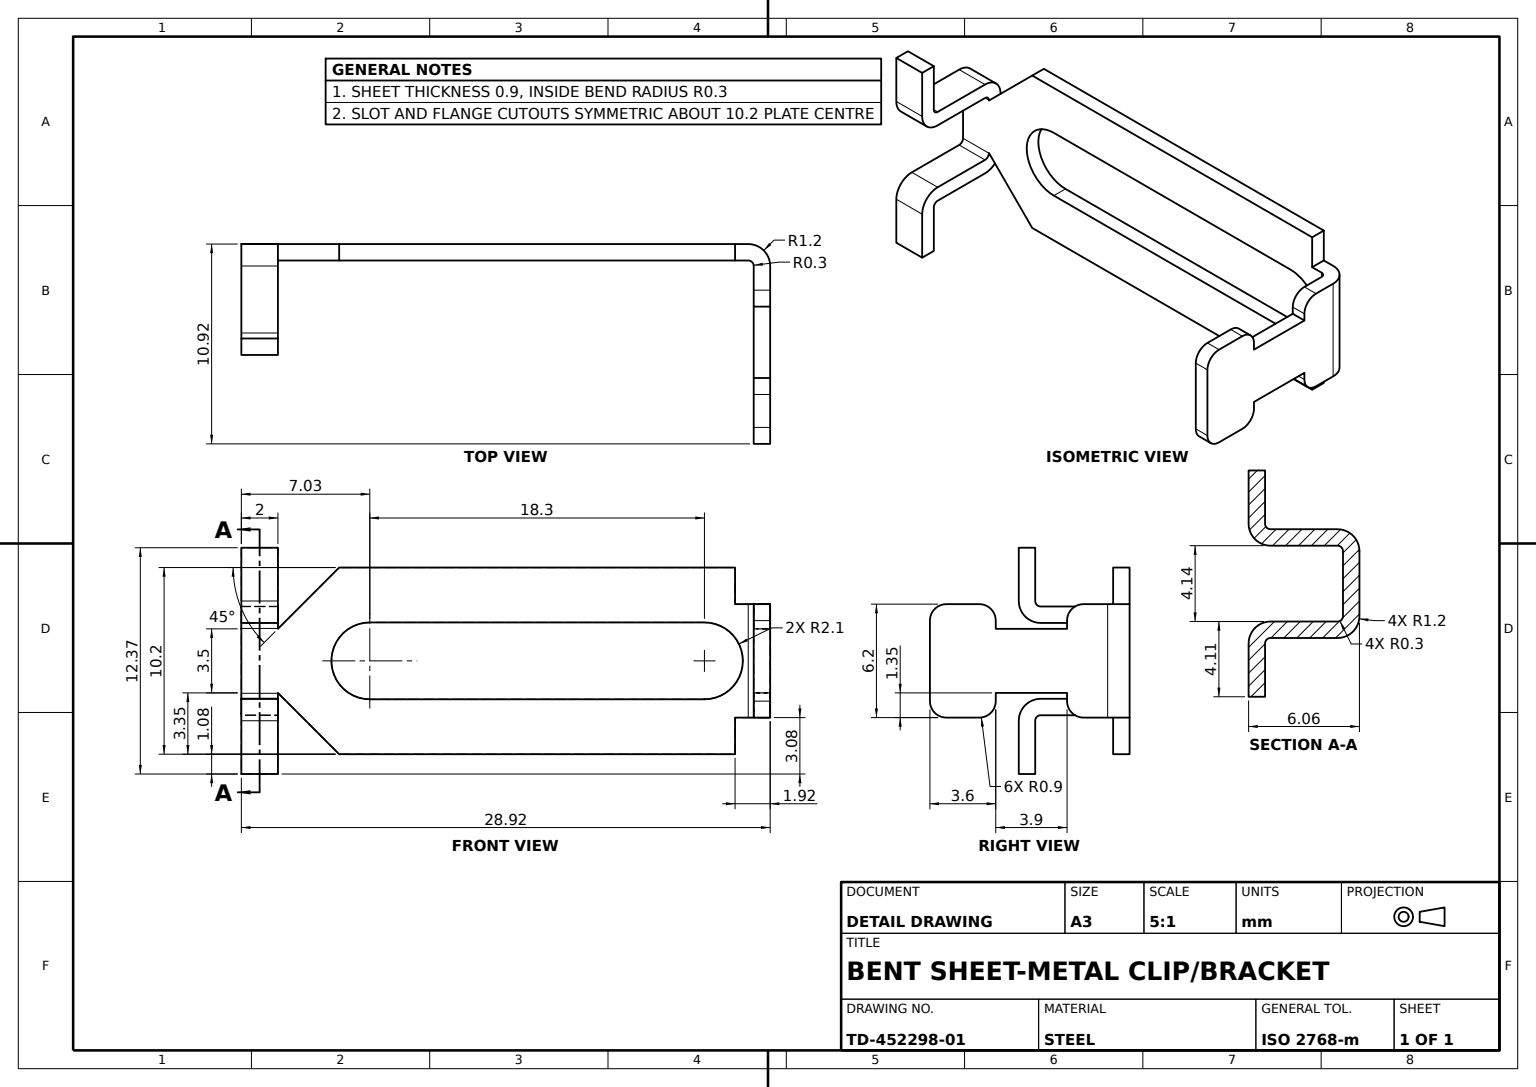
solid
v1 (-1.567146,-5.610951,16.175)
v2 (-1.567146,-4.710951,16.175)
e1 v1 v2 LINE
v3 (-1.867146,-4.410951,16.175)
e2 v3 v2 CIRCLE(AX(P(-1.567146,-4.410951,16.175),D(0,0,1),D(1,0,0)),0.3)
v4 (-2.767146,-4.410951,16.175)
e3 v4 v3 LINE
e4 v4 v1 CIRCLE(AX(P(-1.567146,-4.410951,16.175),D(0,0,1),D(-1,0,0)),1.2)
face PLANE(AX(P(-1.567146,-4.410951,16.175),D(0,0,-1),D(-1,0,0))) rev [e1 -e2 -e3 e4]
v5 (0.652854,-4.839049,-11.845)
v6 (0.652854,-4.839049,-12.745)
e5 v5 v6 LINE
v7 (0.652854,-4.389049,-12.745)
e6 v7 v6 LINE
v8 (0.652854,-4.389049,-11.845)
e7 v7 v8 LINE
e8 v8 v5 LINE
face PLANE(AX(P(0.652854,-5.739049,-12.745),D(-1,0,0),D(0,0,-1))) rev [e5 -e6 e7 e8]
v9 (4.552854,-0.439049,-12.745)
v10 (5.452854,0.460951,-12.745)
e9 v9 v10 CIRCLE(AX(P(5.452854,-0.439049,-12.745),D(0,0,-1),D(-1,0,0)),0.9)
v11 (4.552854,-0.439049,-11.845)
e10 v11 v9 LINE
v12 (5.452854,0.460951,-11.845)
e11 v12 v11 CIRCLE(AX(P(5.452854,-0.439049,-11.845),D(0,0,1),D(-1,0,0)),0.9)
e12 v10 v12 LINE
face CYL(AX(P(5.452854,-0.439049,-12.745),D(0,0,1),D(0,-1,0)),0.9) [-e9 -e10 -e11 -e12]
v13 (4.552854,-0.889049,-11.845)
e13 v13 v11 LINE
v14 (0.652854,-0.889049,-11.845)
e14 v14 v13 LINE
v15 (0.652854,-0.439049,-11.845)
e15 v15 v14 LINE
v16 (-0.247146,0.460951,-11.845)
e16 v15 v16 CIRCLE(AX(P(-0.247146,-0.439049,-11.845),D(0,0,1),D(-1,0,0)),0.9)
v17 (-1.567146,0.460951,-11.845)
e17 v17 v16 LINE
v18 (-1.567146,-5.739049,-11.845)
e18 v18 v17 LINE
v19 (-0.247146,-5.739049,-11.845)
e19 v19 v18 LINE
e20 v19 v5 CIRCLE(AX(P(-0.247146,-4.839049,-11.845),D(0,0,1),D(-1,0,0)),0.9)
v20 (4.552854,-4.389049,-11.845)
e21 v20 v8 LINE
v21 (4.552854,-4.839049,-11.845)
e22 v21 v20 LINE
v22 (5.452854,-5.739049,-11.845)
e23 v21 v22 CIRCLE(AX(P(5.452854,-4.839049,-11.845),D(0,0,1),D(-1,0,0)),0.9)
v23 (7.252854,-5.739049,-11.845)
e24 v23 v22 LINE
v24 (8.152854,-4.839049,-11.845)
e25 v23 v24 CIRCLE(AX(P(7.252854,-4.839049,-11.845),D(0,0,1),D(-1,0,0)),0.9)
v25 (8.152854,-0.439049,-11.845)
e26 v25 v24 LINE
v26 (7.252854,0.460951,-11.845)
e27 v25 v26 CIRCLE(AX(P(7.252854,-0.439049,-11.845),D(0,0,1),D(-1,0,0)),0.9)
e28 v12 v26 LINE
face PLANE(AX(P(-2.317146,-2.639049,-11.845),D(0,0,1),D(-1,0,0))) [-e13 -e14 -e15 e16 -e17 -e18 -e19 e20 -e8 -e21 -e22 e23 -e24 e25 -e26 e27 -e28 e11]
v27 (7.252854,0.460951,-12.745)
v28 (8.152854,-0.439049,-12.745)
e29 v27 v28 CIRCLE(AX(P(7.252854,-0.439049,-12.745),D(0,0,-1),D(-1,0,0)),0.9)
e30 v26 v27 LINE
e31 v28 v25 LINE
face CYL(AX(P(7.252854,-0.439049,-12.745),D(0,0,1),D(-1,0,0)),0.9) [-e29 -e30 -e27 -e31]
v29 (-1.867146,0.460951,-11.545)
e32 v17 v29 CIRCLE(AX(P(-1.567146,0.460951,-11.545),D(0,1,0),D(-1,0,0)),0.3)
v30 (-1.867146,-5.739049,-11.545)
e33 v29 v30 LINE
e34 v30 v18 CIRCLE(AX(P(-1.567146,-5.739049,-11.545),D(0,-1,0),D(1,0,0)),0.3)
face CYL(AX(P(-1.567146,-9.013836,-11.545),D(0,1,0),D(-1,0,0)),0.3) rev [e18 e32 e33 e34]
v31 (2.393806,0.632854,16.175)
v32 (3.293806,0.632854,16.175)
e35 v31 v32 LINE
v33 (3.293806,3.543806,16.175)
e36 v33 v32 LINE
v34 (2.393806,3.543806,16.175)
e37 v34 v33 LINE
e38 v34 v31 LINE
face PLANE(AX(P(3.293806,-5.406194,16.175),D(0,0,-1),D(0,-1,0))) rev [e35 -e36 -e37 e38]
v35 (-1.567146,0.460951,-12.745)
v36 (-2.767146,0.460951,-11.545)
e39 v35 v36 CIRCLE(AX(P(-1.567146,0.460951,-11.545),D(0,1,0),D(-1,0,0)),1.2)
e40 v29 v36 LINE
e41 v17 v35 LINE
face PLANE(AX(P(-1.567146,0.460951,-11.545),D(0,-1,0),D(1,0,0))) rev [e39 -e40 -e32 e41]
v37 (-2.767146,-0.539049,-9.15)
v38 (-2.767146,-0.539049,9.15)
e42 v37 v38 LINE
v39 (-1.867146,-0.539049,-9.15)
e43 v37 v39 LINE
v40 (-1.867146,-0.539049,9.15)
e44 v39 v40 LINE
e45 v38 v40 LINE
face PLANE(AX(P(-1.867146,-0.539049,-9.15),D(0,-1,0),D(0,0,1))) [-e42 e43 e44 -e45]
v41 (4.552854,-0.889049,-12.745)
e46 v41 v13 LINE
v42 (0.652854,-0.889049,-12.745)
e47 v42 v41 LINE
e48 v42 v14 LINE
face PLANE(AX(P(4.552854,-0.889049,-12.745),D(0,-1,0),D(0,0,-1))) rev [e14 -e46 -e47 e48]
v43 (2.093806,0.332854,14.175)
v44 (2.393806,0.632854,14.175)
e49 v43 v44 CIRCLE(AX(P(2.093806,0.632854,14.175),D(0,0,1),D(0,-1,0)),0.3)
v45 (2.093806,0.332854,16.175)
e50 v43 v45 LINE
e51 v31 v45 CIRCLE(AX(P(2.093806,0.632854,16.175),D(0,0,-1),D(0,-1,0)),0.3)
e52 v44 v31 LINE
face CYL(AX(P(2.093806,0.632854,12.685439),D(0,0,1),D(0,-1,0)),0.3) rev [-e49 e50 -e51 -e52]
v46 (2.093806,-5.610951,16.175)
e53 v1 v46 LINE
v47 (2.093806,-4.710951,16.175)
e54 v46 v47 LINE
e55 v2 v47 LINE
face PLANE(AX(P(-6.267146,-4.710951,16.175),D(0,0,-1),D(1,0,0))) rev [e53 e54 -e55 -e1]
v48 (3.293806,0.632854,14.175)
e56 v48 v44 LINE
v49 (2.093806,-0.567146,14.175)
e57 v49 v48 CIRCLE(AX(P(2.093806,0.632854,14.175),D(0,0,1),D(0,-1,0)),1.2)
e58 v49 v43 LINE
face PLANE(AX(P(2.093806,0.632854,14.175),D(0,0,-1),D(0,1,0))) [-e56 -e57 e58 e49]
v50 (3.293806,-5.910951,14.175)
v51 (3.293806,-5.910951,16.175)
e59 v50 v51 LINE
v52 (3.293806,-8.821903,16.175)
e60 v51 v52 LINE
v53 (3.293806,-8.821903,14.175)
e61 v52 v53 LINE
e62 v53 v50 LINE
face PLANE(AX(P(3.293806,1.878097,0),D(-1,0,0),D(0,0,-1))) rev [e59 e60 e61 e62]
v54 (-2.767146,-7.739049,-10.825)
v55 (-2.767146,-5.739049,-10.825)
e63 v54 v55 LINE
v56 (-1.867146,-5.739049,-10.825)
e64 v55 v56 LINE
v57 (-1.867146,-7.739049,-10.825)
e65 v57 v56 LINE
e66 v54 v57 LINE
face PLANE(AX(P(-1.867146,-5.739049,-10.825),D(0,0,1),D(0,1,0))) rev [e63 e64 -e65 -e66]
v58 (8.152854,-4.839049,-12.745)
v59 (7.252854,-5.739049,-12.745)
e67 v58 v59 CIRCLE(AX(P(7.252854,-4.839049,-12.745),D(0,0,-1),D(-1,0,0)),0.9)
e68 v24 v58 LINE
e69 v59 v23 LINE
face CYL(AX(P(7.252854,-4.839049,-12.745),D(0,0,1),D(-1,0,0)),0.9) [-e67 -e68 -e25 -e69]
v60 (-1.567146,-0.567146,14.175)
e70 v60 v49 LINE
v61 (2.093806,-0.567146,16.175)
e71 v49 v61 LINE
v62 (-1.567146,-0.567146,16.175)
e72 v61 v62 LINE
e73 v60 v62 LINE
face PLANE(AX(P(-4.517146,-0.567146,0),D(0,1,0),D(0,0,-1))) rev [e70 e71 e72 -e73]
v63 (-1.867146,-0.867146,16.175)
e74 v63 v3 LINE
v64 (-2.767146,-0.867146,16.175)
e75 v64 v63 LINE
e76 v64 v4 LINE
face PLANE(AX(P(-1.867146,-0.889049,16.175),D(0,0,-1),D(0,-1,0))) rev [-e74 -e75 e76 e3]
v65 (-1.567146,0.332854,14.175)
e77 v60 v65 LINE
v66 (-1.867146,-0.867146,14.175)
e78 v66 v60 CIRCLE(AX(P(-1.567146,-0.867146,14.175),D(0,0,-1),D(-1,0,0)),0.3)
v67 (-2.767146,-0.867146,14.175)
e79 v66 v67 LINE
e80 v67 v65 CIRCLE(AX(P(-1.567146,-0.867146,14.175),D(0,0,-1),D(1,0,0)),1.2)
face PLANE(AX(P(-1.567146,-0.867146,14.175),D(0,0,1),D(1,0,0))) rev [-e77 -e78 e79 e80]
v68 (2.393806,-5.910951,16.175)
v69 (2.393806,-8.821903,16.175)
e81 v68 v69 LINE
e82 v69 v52 LINE
e83 v68 v51 LINE
face PLANE(AX(P(3.293806,3.628097,16.175),D(0,0,-1),D(0,-1,0))) rev [e81 e82 -e60 -e83]
v70 (5.452854,-5.739049,-12.745)
e84 v22 v70 LINE
e85 v59 v70 LINE
face PLANE(AX(P(-1.867146,-5.739049,-12.745),D(0,1,0),D(0,0,1))) rev [e24 e84 -e85 e69]
e86 v10 v27 LINE
face PLANE(AX(P(8.152854,0.460951,-12.745),D(0,-1,0),D(0,0,-1))) rev [-e86 e12 e28 e30]
v71 (2.393806,-8.821903,14.175)
v72 (2.393806,-5.910951,14.175)
e87 v71 v72 LINE
e88 v69 v71 LINE
e89 v72 v68 LINE
face PLANE(AX(P(2.393806,1.878097,0),D(-1,0,0),D(0,0,-1))) [-e87 -e88 -e81 -e89]
v73 (4.552854,-4.389049,-12.745)
e90 v73 v7 LINE
e91 v73 v20 LINE
face PLANE(AX(P(4.552854,-4.389049,-12.745),D(0,1,0),D(0,0,1))) rev [-e7 -e90 e91 e21]
v74 (-2.767146,2.460951,10.825)
v75 (-1.867146,2.460951,10.825)
e92 v74 v75 LINE
v76 (-1.867146,2.460951,-10.825)
e93 v76 v75 LINE
v77 (-2.767146,2.460951,-10.825)
e94 v77 v76 LINE
e95 v77 v74 LINE
face PLANE(AX(P(-1.867146,2.460951,-10.825),D(0,-1,0),D(0,0,1))) rev [e92 -e93 -e94 e95]
v78 (-2.767146,-4.739049,9.15)
e96 v38 v78 CIRCLE(AX(P(-2.767146,-2.639049,9.15),D(1,0,0),D(0,0,1)),2.1)
v79 (-1.867146,-4.739049,9.15)
e97 v40 v79 CIRCLE(AX(P(-1.867146,-2.639049,9.15),D(1,0,0),D(0,0,1)),2.1)
e98 v78 v79 LINE
face CYL(AX(P(-1.867146,-2.639049,9.15),D(-1,0,0),D(0,0,-1)),2.1) rev [-e96 e45 e97 -e98]
e99 v32 v61 CIRCLE(AX(P(2.093806,0.632854,16.175),D(0,0,-1),D(0,1,0)),1.2)
e100 v45 v61 LINE
face PLANE(AX(P(2.093806,0.632854,16.175),D(0,0,1),D(0,-1,0))) [-e99 -e35 e51 e100]
v80 (-1.567146,-5.610951,14.175)
v81 (-2.767146,-4.410951,14.175)
e101 v80 v81 CIRCLE(AX(P(-1.567146,-4.410951,14.175),D(0,0,-1),D(-1,0,0)),1.2)
e102 v80 v1 LINE
e103 v81 v4 LINE
face CYL(AX(P(-1.567146,-4.410951,17.664561),D(0,0,-1),D(-1,0,0)),1.2) [-e101 e102 -e4 -e103]
v82 (-1.567146,-4.710951,14.175)
e104 v82 v80 LINE
v83 (2.093806,-4.710951,14.175)
e105 v83 v82 LINE
v84 (2.093806,-5.610951,14.175)
e106 v83 v84 LINE
e107 v84 v80 LINE
face PLANE(AX(P(-2.767146,-5.610951,14.175),D(0,0,-1),D(-1,0,0))) [-e104 -e105 e106 e107]
v85 (-2.767146,-5.739049,-11.545)
e108 v36 v85 LINE
v86 (-1.567146,-5.739049,-12.745)
e109 v35 v86 LINE
e110 v85 v86 CIRCLE(AX(P(-1.567146,-5.739049,-11.545),D(0,-1,0),D(-1,0,0)),1.2)
face CYL(AX(P(-1.567146,-9.013836,-11.545),D(0,1,0),D(-1,0,0)),1.2) [-e108 -e39 e109 -e110]
v87 (-2.767146,-7.739049,10.825)
e111 v87 v54 LINE
v88 (-1.867146,-7.739049,10.825)
e112 v88 v57 LINE
e113 v87 v88 LINE
face PLANE(AX(P(-1.867146,-7.739049,-10.825),D(0,1,0),D(0,0,-1))) rev [e111 e66 -e112 -e113]
v89 (-2.767146,-4.739049,-9.15)
v90 (-2.767146,-2.639049,-11.25)
e114 v89 v90 CIRCLE(AX(P(-2.767146,-2.639049,-9.15),D(1,0,0),D(0,0,1)),2.1)
e115 v90 v37 CIRCLE(AX(P(-2.767146,-2.639049,-9.15),D(1,0,0),D(0,0,1)),2.1)
e116 v78 v89 LINE
v91 (-2.767146,-4.389049,14.175)
e117 v91 v87 LINE
e118 v81 v91 LINE
e119 v67 v64 LINE
v92 (-2.767146,-0.889049,14.175)
e120 v92 v67 LINE
e121 v74 v92 LINE
v93 (-2.767146,0.460951,-10.825)
e122 v93 v77 LINE
e123 v36 v93 LINE
e124 v55 v85 LINE
face PLANE(AX(P(-2.767146,-2.639049,0),D(-1,0,0),D(0,0,-1))) [e114 e115 e42 e96 e116] [-e117 -e118 e103 -e76 -e119 -e120 -e121 -e95 -e122 -e123 e108 -e124 -e63 -e111]
v94 (4.552854,-4.839049,-12.745)
e125 v94 v21 LINE
e126 v70 v94 CIRCLE(AX(P(5.452854,-4.839049,-12.745),D(0,0,-1),D(-1,0,0)),0.9)
face CYL(AX(P(5.452854,-4.839049,-12.745),D(0,0,1),D(0,-1,0)),0.9) [-e84 -e23 -e125 -e126]
e127 v83 v47 LINE
e128 v82 v2 LINE
face PLANE(AX(P(-4.517146,-4.710951,0),D(0,-1,0),D(0,0,-1))) rev [-e127 e105 e128 e55]
v95 (-1.867146,-4.389049,14.175)
e129 v91 v95 LINE
v96 (-1.867146,-4.410951,14.175)
e130 v96 v95 LINE
e131 v96 v81 LINE
face PLANE(AX(P(-2.767146,-4.389049,14.175),D(0,0,-1),D(0,1,0))) [e129 -e130 e131 e118]
e132 v47 v51 CIRCLE(AX(P(2.093806,-5.910951,16.175),D(0,0,-1),D(0,-1,0)),1.2)
e133 v46 v68 CIRCLE(AX(P(2.093806,-5.910951,16.175),D(0,0,-1),D(0,-1,0)),0.3)
face PLANE(AX(P(2.093806,-5.910951,16.175),D(0,0,1),D(0,1,0))) [-e132 -e54 e133 e83]
v97 (-0.247146,-5.739049,-12.745)
e134 v97 v19 LINE
e135 v6 v97 CIRCLE(AX(P(-0.247146,-4.839049,-12.745),D(0,0,-1),D(-1,0,0)),0.9)
face CYL(AX(P(-0.247146,-4.839049,-12.745),D(0,0,1),D(0,-1,0)),0.9) [-e134 -e135 -e5 -e20]
v98 (-1.567146,0.332854,16.175)
e136 v65 v98 LINE
e137 v98 v64 CIRCLE(AX(P(-1.567146,-0.867146,16.175),D(0,0,1),D(1,0,0)),1.2)
face CYL(AX(P(-1.567146,-0.867146,12.685439),D(0,0,1),D(1,0,0)),1.2) [-e136 -e80 e119 -e137]
e138 v30 v85 LINE
e139 v56 v30 LINE
face PLANE(AX(P(-1.867146,-5.739049,-12.745),D(0,1,0),D(0,0,-1))) rev [-e64 e124 -e138 -e139]
e140 v48 v32 LINE
face CYL(AX(P(2.093806,0.632854,12.685439),D(0,0,1),D(0,-1,0)),1.2) [-e71 e57 e140 e99]
v99 (-1.867146,0.460951,-10.825)
e141 v93 v99 LINE
e142 v99 v76 LINE
face PLANE(AX(P(-1.867146,2.460951,-10.825),D(0,0,1),D(0,1,0))) rev [-e141 e122 e94 -e142]
v100 (2.393806,3.543806,14.175)
e143 v100 v34 LINE
e144 v44 v100 LINE
face PLANE(AX(P(2.393806,-7.156194,0),D(-1,0,0),D(0,0,-1))) [e52 -e38 -e143 -e144]
v101 (-0.247146,0.460951,-12.745)
e145 v35 v101 LINE
e146 v16 v101 LINE
face PLANE(AX(P(8.152854,0.460951,-12.745),D(0,-1,0),D(0,0,-1))) rev [-e145 -e41 e17 e146]
e147 v50 v83 CIRCLE(AX(P(2.093806,-5.910951,14.175),D(0,0,1),D(0,1,0)),1.2)
face CYL(AX(P(2.093806,-5.910951,17.664561),D(0,0,-1),D(0,-1,0)),1.2) [e127 e132 -e59 e147]
v102 (0.652854,-0.439049,-12.745)
e148 v102 v42 LINE
e149 v102 v15 LINE
face PLANE(AX(P(0.652854,0.460951,-12.745),D(-1,0,0),D(0,-1,0))) rev [-e148 e149 e15 -e48]
e150 v50 v72 LINE
e151 v71 v53 LINE
face PLANE(AX(P(2.393806,0.128097,14.175),D(0,0,-1),D(0,1,0))) [-e150 -e62 -e151 e87]
e152 v41 v9 LINE
face PLANE(AX(P(4.552854,0.460951,-12.745),D(1,0,0),D(0,0,1))) rev [-e152 e46 e13 e10]
e153 v101 v102 CIRCLE(AX(P(-0.247146,-0.439049,-12.745),D(0,0,-1),D(-1,0,0)),0.9)
face CYL(AX(P(-0.247146,-0.439049,-12.745),D(0,0,1),D(0,-1,0)),0.9) [-e16 -e149 -e153 -e146]
face PLANE(AX(P(2.393806,-8.821903,16.175),D(0,-1,0),D(0,0,-1))) [-e61 -e82 e88 e151]
e154 v18 v86 LINE
face PLANE(AX(P(-1.567146,-5.739049,-11.545),D(0,1,0),D(-1,0,0))) rev [e110 -e154 -e34 e138]
e155 v84 v46 LINE
face PLANE(AX(P(-4.517146,-5.610951,0),D(0,-1,0),D(0,0,-1))) [e155 -e53 -e102 -e107]
v103 (3.293806,3.543806,14.175)
e156 v103 v33 LINE
e157 v100 v103 LINE
face PLANE(AX(P(2.393806,3.543806,14.175),D(0,1,0),D(0,0,1))) [-e156 -e157 e143 e37]
e158 v62 v63 CIRCLE(AX(P(-1.567146,-0.867146,16.175),D(0,0,1),D(1,0,0)),0.3)
e159 v98 v62 LINE
face PLANE(AX(P(-1.567146,-0.867146,16.175),D(0,0,-1),D(-1,0,0))) rev [e137 e75 -e158 -e159]
e160 v72 v84 CIRCLE(AX(P(2.093806,-5.910951,14.175),D(0,0,1),D(0,-1,0)),0.3)
face PLANE(AX(P(2.093806,-5.910951,14.175),D(0,0,-1),D(0,-1,0))) [-e106 -e147 e150 e160]
e161 v82 v96 CIRCLE(AX(P(-1.567146,-4.410951,14.175),D(0,0,-1),D(-1,0,0)),0.3)
e162 v96 v3 LINE
face CYL(AX(P(-1.567146,-4.410951,17.664561),D(0,0,-1),D(-1,0,0)),0.3) rev [e2 -e128 e161 e162]
v104 (-1.867146,-0.889049,14.175)
e163 v104 v66 LINE
e164 v92 v104 LINE
face PLANE(AX(P(-2.767146,-0.889049,14.175),D(0,0,-1),D(0,1,0))) [-e79 -e163 -e164 e120]
e165 v94 v73 LINE
face PLANE(AX(P(4.552854,-5.739049,-12.745),D(1,0,0),D(0,1,0))) rev [-e91 -e165 e125 e22]
e166 v45 v98 LINE
face PLANE(AX(P(-2.767146,-0.567146,16.175),D(0,0,-1),D(-1,0,0))) rev [-e100 e166 e159 -e72]
face PLANE(AX(P(-1.567146,-4.410951,14.175),D(0,0,1),D(1,0,0))) rev [e101 -e131 -e161 e104]
e167 v48 v103 LINE
face PLANE(AX(P(2.393806,-5.406194,14.175),D(0,0,-1),D(0,1,0))) [e56 e144 e157 -e167]
e168 v97 v86 LINE
face PLANE(AX(P(-1.867146,-5.739049,-12.745),D(0,1,0),D(0,0,1))) rev [e134 e19 e154 -e168]
e169 v29 v99 LINE
face PLANE(AX(P(-1.867146,0.460951,-10.825),D(0,-1,0),D(0,0,1))) rev [e123 e141 -e169 e40]
v105 (-1.867146,-2.639049,-11.25)
e170 v105 v39 CIRCLE(AX(P(-1.867146,-2.639049,-9.15),D(1,0,0),D(0,0,-1)),2.1)
v106 (-1.867146,-4.739049,-9.15)
e171 v106 v105 CIRCLE(AX(P(-1.867146,-2.639049,-9.15),D(1,0,0),D(0,0,-1)),2.1)
e172 v79 v106 LINE
e173 v75 v104 LINE
e174 v66 v63 LINE
e175 v95 v88 LINE
face PLANE(AX(P(-1.867146,-2.639049,0),D(-1,0,0),D(0,0,-1))) rev [-e44 -e170 -e171 -e172 -e97] [e142 e93 e173 e163 e174 e74 -e162 e130 e175 e112 e65 e139 -e33 e169]
e176 v105 v90 LINE
face CYL(AX(P(-1.867146,-2.639049,-9.15),D(-1,0,0),D(0,0,-1)),2.1) rev [-e176 e170 -e43 -e115]
e177 v28 v58 LINE
face PLANE(AX(P(8.152854,-5.739049,-12.745),D(-1,0,0),D(0,0,-1))) rev [-e177 e31 e26 e68]
face PLANE(AX(P(-2.317146,-2.639049,-12.745),D(0,0,1),D(-1,0,0))) rev [e29 e177 e67 e85 e126 e165 e90 e6 e135 e168 -e109 e145 e153 e148 e47 e152 e9 e86]
e178 v65 v43 LINE
face PLANE(AX(P(-2.767146,0.332854,14.175),D(0,0,-1),D(1,0,0))) [-e58 -e70 e77 e178]
face CYL(AX(P(2.093806,-5.910951,17.664561),D(0,0,-1),D(0,-1,0)),0.3) rev [e89 -e133 -e155 -e160]
face PLANE(AX(P(3.293806,-7.156194,0),D(-1,0,0),D(0,0,-1))) rev [-e140 e167 e156 e36]
face PLANE(AX(P(-1.867146,2.460951,10.825),D(0,-0.707106781,-0.707106781),D(0,-0.707106781,0.707106781))) rev [-e173 -e92 e121 e164]
e179 v89 v106 LINE
face PLANE(AX(P(-1.867146,-4.739049,-9.15),D(0,1,0),D(0,0,-1))) [e98 e172 -e179 -e116]
face PLANE(AX(P(-4.517146,0.332854,0),D(0,1,0),D(0,0,-1))) [-e178 e136 -e166 -e50]
face CYL(AX(P(-1.867146,-2.639049,-9.15),D(-1,0,0),D(0,0,-1)),2.1) rev [-e114 e179 e171 e176]
face PLANE(AX(P(-1.867146,-4.389049,14.175),D(0,0.707106781,-0.707106781),D(0,-0.707106781,-0.707106781))) rev [-e175 -e129 e117 e113]
face CYL(AX(P(-1.567146,-0.867146,12.685439),D(0,0,1),D(1,0,0)),0.3) rev [e78 e73 e158 -e174]
